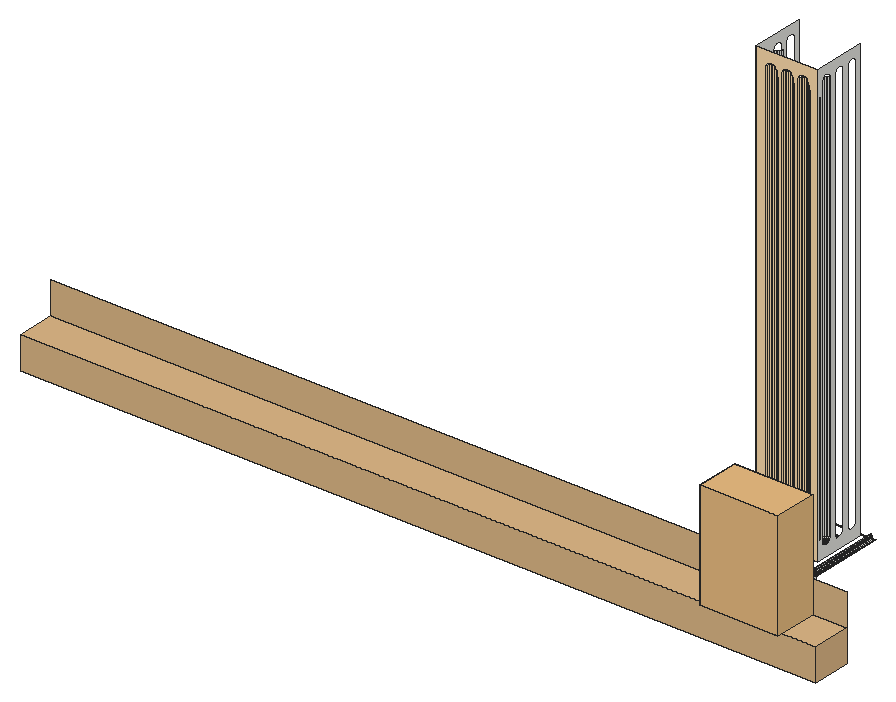
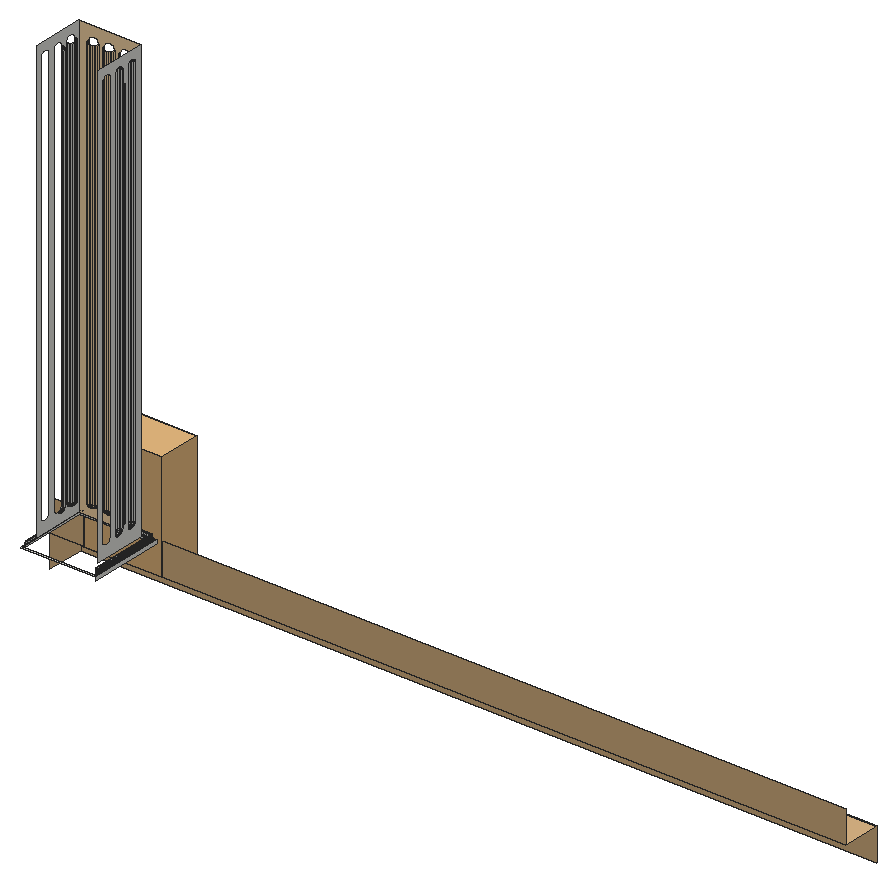
# SketchUp Ruby script. Lengths in inches.
U = 1.inch
M = Sketchup.active_model
def pt(a) = Geom::Point3d.new(a.map { |v| v * U })
def face(e, loops, mat)
  f = e.add_face(loops[0].map { |a| pt(a) })
  loops[1..].each { |l| e.add_face(l.map { |a| pt(a) }).erase! }
  f.material = f.back_material = mat if mat
  f
end
# faces: each face lists its corners as indices into pts; further lists are holes
def faces(e, pts, list, mat = nil) = list.each { |f| face(e, (f[0].is_a?(Array) ? f : [f]).map { |l| l.map { |i| pts[i] } }, mat) }
# xy, xz, yz: faces in a plane at the given z, y or x. An outline is a flat list of corners, or four numbers for a rectangle; further outlines are holes
def ring(l) = l.size == 4 ? [[l[0], l[1]], [l[2], l[1]], [l[2], l[3]], [l[0], l[3]]] : l.each_slice(2).to_a
def flat(e, list, mat, &to3) = list.each { |f| face(e, (f[0].is_a?(Array) ? f : [f]).map { |l| ring(l).map { |u, v| to3.(u, v) } }, mat) }
def xy(e, z, list, mat = nil) = flat(e, list, mat) { |x, y| [x, y, z] }
def xz(e, y, list, mat = nil) = flat(e, list, mat) { |x, z| [x, y, z] }
def yz(e, x, list, mat = nil) = flat(e, list, mat) { |y, z| [x, y, z] }
def lines(e, pts, list) = list.each { |a, b| e.add_line(pt(pts[a]), pt(pts[b])) }
# prism: a flat outline (further loops are holes) pulled along v
def prism(e, loops, v, mat = nil)
  f = face(e, loops, mat); d = Geom::Vector3d.new(v.map { |x| x * U })
  f.pushpull(f.normal.samedirection?(d) ? d.length : -d.length)
end
def box(e, o, s, mat = nil) = prism(e, [[o, [o[0] + s[0], o[1], o[2]], [o[0] + s[0], o[1] + s[1], o[2]], [o[0], o[1] + s[1], o[2]]]], [0, 0, s[2]], mat)
def at(x, y, z, deg = 0) = Geom::Transformation.translation(pt([x, y, z])) * Geom::Transformation.rotation(ORIGIN, Z_AXIS, deg.degrees)
def axes(o, x, y, z) = Geom::Transformation.new([*x, 0, *y, 0, *z, 0, *pt(o).to_a, 1])
def part(name) = M.definitions.add(name)
# library, detail: a bought-in or finely detailed component or shape, given as its bounding box
def library(name, o, s) = part(name).tap { |d| box(d.entities, o, s) }
def detail(e, o, s) = box(e.add_group.entities, o, s)
def put(e, d, t, mat = nil) = e.add_instance(d, t).tap { |i| i.material = mat if mat }
def group(e, t, mat = nil) = e.add_group.tap { |g| g.transformation = t; g.material = mat if mat }.entities
root = M.entities
M.materials.add("[0033_NavajoWhite]").color = [255, 222, 173]
M.materials.add("[0036_BurlyWood]").color = [222, 184, 135]
c1 = library("Flower+pot",[-3.29,-4.11,0],[8.25,8.08,16.09])
xy(root,6,[[103.43,0,251.04,7.125]],"[0036_BurlyWood]")
xy(root,12.13,[[[230.94,7.58,244.97,21.61],[231.11,7.74,244.81,21.44]]])
xz(root,0,[[103.43,0,251.04,6]],"[0036_BurlyWood]")
xz(root,7.125,[[103.43,6,251.04,12]],"[0036_BurlyWood]")
xz(root,7.58,[[230.94,11.46,244.97,12.13]])
xz(root,8.1,[[231.46,12.13,244.45,13.02],[231.46,13.02,244.45,13.17]])
xz(root,9.67,[[[232.25,13.17,243.67,94.95],[235.01,14.97,234.75,15,234.51,15.09,234.31,15.24,234.15,15.42,234.05,15.64,234.02,15.875,234.02,92.25,234.05,92.48,234.15,92.7,234.31,92.89,234.51,93.03,234.75,93.12,235.01,93.15,235.26,93.12,235.5,93.03,235.7,92.89,235.86,92.7,235.96,92.48,235.99,92.25,235.99,15.875,235.96,15.64,235.86,15.42,235.7,15.24,235.5,15.09,235.26,15],[240.91,14.97,240.66,15,240.42,15.09,240.22,15.24,240.06,15.42,239.96,15.64,239.93,15.875,239.93,92.25,239.96,92.48,240.06,92.7,240.22,92.89,240.42,93.03,240.66,93.12,240.91,93.15,241.17,93.12,241.4,93.03,241.61,92.89,241.76,92.7,241.86,92.48,241.9,92.25,241.9,15.875,241.86,15.64,241.76,15.42,241.61,15.24,241.4,15.09,241.17,15],[237.96,14.97,237.7,15,237.47,15.09,237.26,15.24,237.11,15.42,237.01,15.64,236.97,15.875,236.97,92.25,237.01,92.48,237.11,92.7,237.26,92.89,237.47,93.03,237.7,93.12,237.96,93.15,238.21,93.12,238.45,93.03,238.65,92.89,238.8125,92.7,238.91,92.48,238.94,92.25,238.94,15.875,238.91,15.64,238.8125,15.42,238.65,15.24,238.45,15.09,238.21,15]]],"[0033_NavajoWhite]")
yz(root,230.94,[[7.58,11.46,21.61,12.13]])
yz(root,231.46,[[8.1,12.13,21.09,13.02],[8.1,13.02,21.09,13.17]])
yz(root,232.25,[[[9.67,13.17,19.51,94.95],[17.55,15.23,17.8,15.27,18.04,15.36,18.24,15.5,18.4,15.69,18.5,15.9,18.53,16.14,18.53,92.51,18.5,92.74,18.4,92.96,18.24,93.15,18.04,93.29,17.8,93.38,17.55,93.41,17.29,93.38,17.05,93.29,16.85,93.15,16.69,92.96,16.59,92.74,16.5625,92.51,16.5625,16.14,16.59,15.9,16.69,15.69,16.85,15.5,17.05,15.36,17.29,15.27],[14.59,15.23,14.85,15.27,15.08,15.36,15.29,15.5,15.44,15.69,15.54,15.9,15.58,16.14,15.58,92.51,15.54,92.74,15.44,92.96,15.29,93.15,15.08,93.29,14.85,93.38,14.59,93.41,14.34,93.38,14.1,93.29,13.9,93.15,13.74,92.96,13.64,92.74,13.61,92.51,13.61,16.14,13.64,15.9,13.74,15.69,13.9,15.5,14.1,15.36,14.34,15.27],[11.64,15.23,11.89,15.27,12.13,15.36,12.34,15.5,12.49,15.69,12.59,15.9,12.625,16.14,12.625,92.51,12.59,92.74,12.49,92.96,12.34,93.15,12.13,93.29,11.89,93.38,11.64,93.41,11.39,93.38,11.15,93.29,10.94,93.15,10.79,92.96,10.6875,92.74,10.66,92.51,10.66,16.14,10.6875,15.9,10.79,15.69,10.94,15.5,11.15,15.36,11.39,15.27]]])
yz(root,243.67,[[[9.67,13.17,19.51,94.95],[17.55,15.23,17.29,15.27,17.05,15.36,16.85,15.5,16.69,15.69,16.59,15.9,16.5625,16.14,16.5625,92.51,16.59,92.74,16.69,92.96,16.85,93.15,17.05,93.29,17.29,93.38,17.55,93.41,17.8,93.38,18.04,93.29,18.24,93.15,18.4,92.96,18.5,92.74,18.53,92.51,18.53,16.14,18.5,15.9,18.4,15.69,18.24,15.5,18.04,15.36,17.8,15.27],[14.59,15.23,14.34,15.27,14.1,15.36,13.9,15.5,13.74,15.69,13.64,15.9,13.61,16.14,13.61,92.51,13.64,92.74,13.74,92.96,13.9,93.15,14.1,93.29,14.34,93.38,14.59,93.41,14.85,93.38,15.08,93.29,15.29,93.15,15.44,92.96,15.54,92.74,15.58,92.51,15.58,16.14,15.54,15.9,15.44,15.69,15.29,15.5,15.08,15.36,14.85,15.27],[11.64,15.23,11.39,15.27,11.15,15.36,10.94,15.5,10.79,15.69,10.6875,15.9,10.66,16.14,10.66,92.51,10.6875,92.74,10.79,92.96,10.94,93.15,11.15,93.29,11.39,93.38,11.64,93.41,11.89,93.38,12.13,93.29,12.34,93.15,12.49,92.96,12.59,92.74,12.625,92.51,12.625,16.14,12.59,15.9,12.49,15.69,12.34,15.5,12.13,15.36,11.89,15.27]]])
yz(root,244.45,[[8.1,12.13,21.09,13.02],[8.1,13.02,21.09,13.17]])
yz(root,251.04,[[0,0,7.125,6]],"[0036_BurlyWood]")
p = [[244.81,7.74,12.13],[244.78,7.78,12.15],[231.14,7.78,12.15],[231.11,7.74,12.13],[231.14,21.41,12.15],[231.11,21.44,12.13],
  [244.81,21.44,12.13],[244.78,21.41,12.15],[244.71,7.84,12.2],[231.2,7.84,12.2],[231.2,21.35,12.2],[244.71,21.35,12.2],
  [244.65,7.9,12.27],[231.26,7.9,12.27],[231.26,21.29,12.27],[244.65,21.29,12.27],[244.6,7.95,12.36],[231.32,7.95,12.36],
  [231.32,21.24,12.36],[244.6,21.24,12.36],[244.55,8,12.47],[231.36,8,12.47],[231.36,21.1875,12.47],[244.55,21.1875,12.47],
  [244.52,8.03,12.59],[231.4,8.03,12.59],[231.4,21.15,12.59],[244.52,21.15,12.59],[244.49,8.06,12.73],[231.43,8.06,12.73],
  [231.43,21.12,12.73],[244.49,21.12,12.73],[244.47,8.09,12.87],[231.45,8.09,12.87],[231.45,21.1,12.87],[244.47,21.1,12.87],
  [244.45,8.1,13.02],[231.46,8.1,13.02],[231.46,21.09,13.02],[244.45,21.09,13.02],[234.53,9.8,15.09],[234.51,9.67,15.09],
  [234.75,9.67,15],[234.76,9.74,15],[234.78,9.8,15],[234.58,9.92,15.09],[235.01,9.67,14.97],[234.83,9.85,15],
  [234.88,9.89,15],[234.94,9.92,15],[235.01,9.93,15],[235.25,9.74,15],[235.26,9.67,15],[235.23,9.8,15],
  [235.1875,9.85,15],[235.13,9.89,15],[235.07,9.92,15],[235.48,9.8,15.09],[235.43,9.92,15.09],[235.5,9.67,15.09],
  [237.48,9.8,15.09],[237.47,9.67,15.09],[237.7,9.67,15],[237.71,9.74,15],[237.74,9.8,15],[237.53,9.92,15.09],
  [237.96,9.67,14.97],[237.78,9.85,15],[237.83,9.89,15],[237.89,9.92,15],[237.96,9.93,15],[238.2,9.74,15],
  [238.21,9.67,15],[238.18,9.8,15],[238.14,9.85,15],[238.09,9.89,15],[238.02,9.92,15],[238.45,9.67,15.09],
  [238.43,9.8,15.09],[238.38,9.92,15.09],[240.4375,9.8,15.09],[240.42,9.67,15.09],[240.66,9.67,15],[240.67,9.74,15],
  [240.69,9.8,15],[240.48,9.92,15.09],[240.91,9.67,14.97],[240.73,9.85,15],[240.78,9.89,15],[240.85,9.92,15],
  [240.91,9.93,15],[241.16,9.74,15],[241.17,9.67,15],[241.13,9.8,15],[241.09,9.85,15],[241.04,9.89,15],
  [240.98,9.92,15],[241.39,9.8,15.09],[241.34,9.92,15.09],[241.4,9.67,15.09],[234.66,10.02,15.09],[235.35,10.02,15.09],
  [237.61,10.02,15.09],[238.31,10.02,15.09],[240.5625,10.02,15.09],[241.26,10.02,15.09],[234.76,10.1,15.09],[234.88,10.15,15.09],
  [235.01,10.16,15.09],[235.13,10.15,15.09],[235.25,10.1,15.09],[237.71,10.1,15.09],[237.83,10.15,15.09],[237.96,10.16,15.09],
  [238.2,10.1,15.09],[238.09,10.15,15.09],[240.67,10.1,15.09],[240.78,10.15,15.09],[240.91,10.16,15.09],[241.04,10.15,15.09],
  [241.16,10.1,15.09],[234.33,9.85,15.24],[234.31,9.67,15.24],[235.7,9.67,15.24],[235.68,9.85,15.24],[237.29,9.85,15.24],
  [237.26,9.67,15.24],[238.65,9.67,15.24],[238.63,9.85,15.24],[240.24,9.85,15.24],[240.22,9.67,15.24],[241.61,9.67,15.24],
  [241.58,9.85,15.24],[234.4,10.02,15.24],[235.61,10.02,15.24],[237.36,10.02,15.24],[238.5625,10.02,15.24],[240.31,10.02,15.24],
  [241.51,10.02,15.24],[234.51,10.16,15.24],[235.5,10.16,15.24],[237.47,10.16,15.24],[238.45,10.16,15.24],[240.42,10.16,15.24],
  [241.4,10.16,15.24],[234.66,10.27,15.24],[235.35,10.27,15.24],[237.61,10.27,15.24],[238.31,10.27,15.24],[240.5625,10.27,15.24],
  [241.26,10.27,15.24],[234.83,10.34,15.24],[235.01,10.37,15.24],[235.1875,10.34,15.24],[237.78,10.34,15.24],[237.96,10.37,15.24],
  [238.14,10.34,15.24],[240.73,10.34,15.24],[240.91,10.37,15.24],[241.09,10.34,15.24],[234.18,9.89,15.42],[234.15,9.67,15.42],
  [235.86,9.67,15.42],[235.83,9.89,15.42],[237.14,9.89,15.42],[237.11,9.67,15.42],[238.8125,9.67,15.42],[238.78,9.89,15.42],
  [240.09,9.89,15.42],[240.06,9.67,15.42],[241.76,9.67,15.42],[241.73,9.89,15.42],[234.27,10.1,15.42],[235.74,10.1,15.42],
  [237.22,10.1,15.42],[238.7,10.1,15.42],[240.17,10.1,15.42],[241.65,10.1,15.42],[234.4,10.27,15.42],[235.61,10.27,15.42],
  [237.36,10.27,15.42],[238.5625,10.27,15.42],[240.31,10.27,15.42],[241.51,10.27,15.42],[234.58,10.41,15.42],[235.43,10.41,15.42],
  [237.53,10.41,15.42],[238.38,10.41,15.42],[240.48,10.41,15.42],[241.34,10.41,15.42],[234.78,10.49,15.42],[235.01,10.52,15.42],
  [235.23,10.49,15.42],[237.74,10.49,15.42],[237.96,10.52,15.42],[238.18,10.49,15.42],[240.69,10.49,15.42],[240.91,10.52,15.42],
  [241.13,10.49,15.42],[232.32,11.39,15.27],[232.25,11.64,15.23],[232.25,11.39,15.27],[232.38,11.42,15.27],[232.43,11.46,15.27],
  [243.6,11.39,15.27],[243.67,11.64,15.23],[243.54,11.42,15.27],[243.49,11.46,15.27],[243.67,11.39,15.27],[232.47,11.51,15.27],
  [232.5,11.57,15.27],[243.45,11.51,15.27],[243.42,11.57,15.27],[232.5,11.64,15.27],[232.5,11.71,15.27],[232.47,11.77,15.27],
  [232.43,11.82,15.27],[232.38,11.86,15.27],[232.32,11.89,15.27],[232.25,11.89,15.27],[243.41,11.64,15.27],[243.42,11.71,15.27],
  [243.45,11.77,15.27],[243.49,11.82,15.27],[243.54,11.86,15.27],[243.6,11.89,15.27],[243.67,11.89,15.27],[232.32,14.35,15.27],
  [232.25,14.59,15.23],[232.25,14.34,15.27],[232.38,14.37,15.27],[243.6,14.35,15.27],[243.67,14.59,15.23],[243.54,14.37,15.27],
  [243.67,14.34,15.27],[232.43,14.41,15.27],[232.47,14.47,15.27],[243.49,14.41,15.27],[243.45,14.47,15.27],[232.5,14.53,15.27],
  [232.5,14.59,15.27],[243.42,14.53,15.27],[243.41,14.59,15.27],[232.25,11.15,15.36],[232.38,11.16,15.36],[243.54,11.16,15.36],
  [243.67,11.15,15.36],[232.5,11.21,15.36],[232.6,11.29,15.36],[243.42,11.21,15.36],[243.32,11.29,15.36],[232.68,11.39,15.36],
  [243.24,11.39,15.36],[232.73,11.51,15.36],[243.19,11.51,15.36],[232.74,11.64,15.36],[243.17,11.64,15.36],[232.73,11.77,15.36],
  [243.19,11.77,15.36],[232.68,11.89,15.36],[243.24,11.89,15.36],[232.6,11.99,15.36],[232.5,12.07,15.36],[243.32,11.99,15.36],
  [243.42,12.07,15.36],[232.38,12.12,15.36],[232.25,12.13,15.36],[243.54,12.12,15.36],[243.67,12.13,15.36],[232.25,14.1,15.36],
  [232.38,14.12,15.36],[232.5,14.17,15.36],[243.54,14.12,15.36],[243.42,14.17,15.36],[243.67,14.1,15.36],[232.6,14.24,15.36],
  [232.68,14.35,15.36],[243.32,14.24,15.36],[243.24,14.35,15.36],[232.73,14.47,15.36],[243.19,14.47,15.36],[232.74,14.59,15.36],
  [243.17,14.59,15.36],[234.09,9.92,15.64],[234.05,9.67,15.64],[235.96,9.67,15.64],[235.92,9.92,15.64],[237.04,9.92,15.64],
  [237.01,9.67,15.64],[238.91,9.67,15.64],[238.875,9.92,15.64],[239.99,9.92,15.64],[239.96,9.67,15.64],[241.86,9.67,15.64],
  [241.83,9.92,15.64],[234.18,10.15,15.64],[235.83,10.15,15.64],[237.14,10.15,15.64],[238.78,10.15,15.64],[240.09,10.15,15.64],
  [241.73,10.15,15.64],[234.33,10.34,15.64],[235.68,10.34,15.64],[237.29,10.34,15.64],[238.63,10.34,15.64],[240.24,10.34,15.64],
  [241.58,10.34,15.64],[234.53,10.49,15.64],[235.48,10.49,15.64],[237.48,10.49,15.64],[238.43,10.49,15.64],[240.4375,10.49,15.64],
  [241.39,10.49,15.64],[234.76,10.59,15.64],[235.25,10.59,15.64],[237.71,10.59,15.64],[238.2,10.59,15.64],[240.67,10.59,15.64],
  [241.16,10.59,15.64],[235.01,10.62,15.64],[237.96,10.62,15.64],[240.91,10.62,15.64],[232.25,10.94,15.5],[232.43,10.97,15.5],
  [243.49,10.97,15.5],[243.67,10.94,15.5],[232.6,11.04,15.5],[232.74,11.15,15.5],[243.32,11.04,15.5],[243.17,11.15,15.5],
  [232.85,11.29,15.5],[243.0625,11.29,15.5],[232.92,11.46,15.5],[242.99,11.46,15.5],[232.95,11.64,15.5],[242.97,11.64,15.5],
  [232.92,11.82,15.5],[242.99,11.82,15.5],[232.85,11.99,15.5],[243.0625,11.99,15.5],[232.74,12.13,15.5],[243.17,12.13,15.5],
  [232.6,12.24,15.5],[243.32,12.24,15.5],[232.43,12.3125,15.5],[232.25,12.34,15.5],[243.49,12.3125,15.5],[243.67,12.34,15.5],
  [232.25,13.9,15.5],[232.43,13.92,15.5],[232.6,13.99,15.5],[243.49,13.92,15.5],[243.32,13.99,15.5],[243.67,13.9,15.5],
  [232.74,14.1,15.5],[243.17,14.1,15.5],[232.85,14.24,15.5],[243.0625,14.24,15.5],[232.92,14.41,15.5],[242.99,14.41,15.5],
  [232.95,14.59,15.5],[242.97,14.59,15.5],[232.25,10.79,15.69],[232.47,10.82,15.69],[232.68,10.9,15.69],[243.45,10.82,15.69],
  [243.24,10.9,15.69],[243.67,10.79,15.69],[232.85,11.04,15.69],[243.0625,11.04,15.69],[232.99,11.21,15.69],[242.93,11.21,15.69],
  [233.07,11.42,15.69],[242.84,11.42,15.69],[233.1,11.64,15.69],[242.81,11.64,15.69],[233.07,11.86,15.69],[242.84,11.86,15.69],
  [232.99,12.07,15.69],[242.93,12.07,15.69],[232.85,12.24,15.69],[243.0625,12.24,15.69],[232.68,12.38,15.69],[243.24,12.38,15.69],
  [232.47,12.46,15.69],[243.45,12.46,15.69],[232.25,12.49,15.69],[243.67,12.49,15.69],[232.25,13.74,15.69],[232.47,13.77,15.69],
  [243.45,13.77,15.69],[243.67,13.74,15.69],[232.68,13.85,15.69],[243.24,13.85,15.69],[232.85,13.99,15.69],[243.0625,13.99,15.69],
  [232.99,14.17,15.69],[242.93,14.17,15.69],[233.07,14.37,15.69],[242.84,14.37,15.69],[233.1,14.59,15.69],[242.81,14.59,15.69],
  [234.05,9.93,15.875],[234.02,9.67,15.875],[235.99,9.67,15.875],[235.96,9.93,15.875],[237.01,9.93,15.875],[236.97,9.67,15.875],
  [238.94,9.67,15.875],[238.91,9.93,15.875],[239.96,9.93,15.875],[239.93,9.67,15.875],[241.9,9.67,15.875],[241.86,9.93,15.875],
  [234.15,10.16,15.875],[235.86,10.16,15.875],[237.11,10.16,15.875],[238.8125,10.16,15.875],[240.06,10.16,15.875],[241.76,10.16,15.875],
  [234.31,10.37,15.875],[235.7,10.37,15.875],[237.26,10.37,15.875],[238.65,10.37,15.875],[240.22,10.37,15.875],[241.61,10.37,15.875],
  [234.51,10.52,15.875],[235.5,10.52,15.875],[237.47,10.52,15.875],[238.45,10.52,15.875],[240.42,10.52,15.875],[241.4,10.52,15.875],
  [234.75,10.62,15.875],[235.26,10.62,15.875],[237.7,10.62,15.875],[238.21,10.62,15.875],[240.66,10.62,15.875],[241.17,10.62,15.875],
  [235.01,10.66,15.875],[237.96,10.66,15.875],[240.91,10.66,15.875],[232.25,10.6875,15.9],[232.5,10.72,15.9],[232.73,10.82,15.9],
  [243.42,10.72,15.9],[243.19,10.82,15.9],[243.67,10.6875,15.9],[232.92,10.97,15.9],[242.99,10.97,15.9],[233.07,11.16,15.9],
  [242.84,11.16,15.9],[233.17,11.39,15.9],[242.75,11.39,15.9],[233.2,11.64,15.9],[242.72,11.64,15.9],[233.17,11.89,15.9],
  [242.75,11.89,15.9],[233.07,12.12,15.9],[242.84,12.12,15.9],[232.92,12.3125,15.9],[242.99,12.3125,15.9],[232.73,12.46,15.9],
  [243.19,12.46,15.9],[232.5,12.56,15.9],[243.42,12.56,15.9],[232.25,12.59,15.9],[243.67,12.59,15.9],[232.25,13.64,15.9],
  [232.5,13.67,15.9],[243.42,13.67,15.9],[243.67,13.64,15.9],[232.73,13.77,15.9],[243.19,13.77,15.9],[232.92,13.92,15.9],
  [242.99,13.92,15.9],[233.07,14.12,15.9],[242.84,14.12,15.9],[233.17,14.35,15.9],[242.75,14.35,15.9],[233.2,14.59,15.9],
  [242.72,14.59,15.9],[234.05,9.93,92.25],[234.02,9.67,92.25],[235.99,9.67,92.25],[235.96,9.93,92.25],[237.01,9.93,92.25],
  [236.97,9.67,92.25],[238.94,9.67,92.25],[238.91,9.93,92.25],[239.96,9.93,92.25],[239.93,9.67,92.25],[241.9,9.67,92.25],
  [241.86,9.93,92.25],[234.15,10.16,92.25],[235.86,10.16,92.25],[237.11,10.16,92.25],[238.8125,10.16,92.25],[240.06,10.16,92.25],
  [241.76,10.16,92.25],[234.31,10.37,92.25],[235.7,10.37,92.25],[237.26,10.37,92.25],[238.65,10.37,92.25],[240.22,10.37,92.25],
  [241.61,10.37,92.25],[234.51,10.52,92.25],[235.5,10.52,92.25],[237.47,10.52,92.25],[238.45,10.52,92.25],[240.42,10.52,92.25],
  [241.4,10.52,92.25],[234.75,10.62,92.25],[235.26,10.62,92.25],[237.7,10.62,92.25],[238.21,10.62,92.25],[240.66,10.62,92.25],
  [241.17,10.62,92.25],[235.01,10.66,92.25],[237.96,10.66,92.25],[240.91,10.66,92.25],[232.25,10.66,16.14],[232.5,10.6875,16.14],
  [232.74,10.79,16.14],[243.41,10.6875,16.14],[243.17,10.79,16.14],[243.67,10.66,16.14],[232.95,10.94,16.14],[242.97,10.94,16.14],
  [233.1,11.15,16.14],[242.81,11.15,16.14],[233.2,11.39,16.14],[242.72,11.39,16.14],[233.23,11.64,16.14],[242.68,11.64,16.14],
  [233.2,11.89,16.14],[242.72,11.89,16.14],[233.1,12.13,16.14],[242.81,12.13,16.14],[232.95,12.34,16.14],[242.97,12.34,16.14],
  [232.74,12.49,16.14],[243.17,12.49,16.14],[232.5,12.59,16.14],[243.41,12.59,16.14],[232.25,12.625,16.14],[243.67,12.625,16.14],
  [232.25,13.61,16.14],[232.5,13.64,16.14],[232.74,13.74,16.14],[243.41,13.64,16.14],[243.17,13.74,16.14],[243.67,13.61,16.14],
  [232.95,13.9,16.14],[242.97,13.9,16.14],[233.1,14.1,16.14],[242.81,14.1,16.14],[233.2,14.34,16.14],[242.72,14.34,16.14],
  [233.23,14.59,16.14],[242.68,14.59,16.14],[232.25,10.66,92.51],[232.5,10.6875,92.51],[232.74,10.79,92.51],[243.17,10.79,92.51],
  [243.41,10.6875,92.51],[243.67,10.66,92.51],[232.95,10.94,92.51],[242.97,10.94,92.51],[233.1,11.15,92.51],[242.81,11.15,92.51],
  [233.2,11.39,92.51],[242.72,11.39,92.51],[233.23,11.64,92.51],[242.68,11.64,92.51],[233.2,11.89,92.51],[242.72,11.89,92.51],
  [233.1,12.13,92.51],[242.81,12.13,92.51],[232.95,12.34,92.51],[242.97,12.34,92.51],[232.74,12.49,92.51],[243.17,12.49,92.51],
  [232.5,12.59,92.51],[243.41,12.59,92.51],[232.25,12.625,92.51],[243.67,12.625,92.51],[232.25,13.61,92.51],[232.5,13.64,92.51],
  [232.74,13.74,92.51],[243.17,13.74,92.51],[243.41,13.64,92.51],[243.67,13.61,92.51],[232.95,13.9,92.51],[242.97,13.9,92.51],
  [233.1,14.1,92.51],[242.81,14.1,92.51],[233.2,14.34,92.51],[242.72,14.34,92.51],[233.23,14.59,92.51],[242.68,14.59,92.51],
  [245.1,7.45,11.45],[245.14,7.41,11.4],[245.18,7.37,11.33]]
faces(root,p,[[0,1,2,3],[2,4,5,3],[0,6,7,1],[1,8,9,2],[9,10,4,2],[1,7,11,8],[8,12,13,9],[13,14,10,9],
  [8,11,15,12],[12,16,17,13],[17,18,14,13],[12,15,19,16],[16,20,21,17],[21,22,18,17],[16,19,23,20],[20,24,25,21],
  [25,26,22,21],[20,23,27,24],[24,28,29,25],[29,30,26,25],[24,27,31,28],[28,32,33,29],[33,34,30,29],[28,31,35,32],
  [32,36,37,33],[37,38,34,33],[32,35,39,36],[199,200,201],[200,199,202],[200,202,203],[204,205,206],[206,205,207],
  [205,204,208],[200,203,209],[200,209,210],[207,205,211],[211,205,212],[200,210,213],[200,213,214],[200,214,215],
  [200,215,216],[200,216,217],[200,217,218],[218,219,200],[212,205,220],[220,205,221],[221,205,222],[222,205,223],
  [223,205,224],[224,205,225],[226,225,205],[227,228,229],[228,227,230],[231,232,233],[232,231,234],[228,230,235],
  [228,235,236],[237,232,238],[233,232,237],[228,236,239],[228,239,240],[238,232,241],[241,232,242],[199,201,243,244],
  [208,204,245,246],[199,244,247,202],[202,247,248,203],[249,206,207,250],[245,204,206,249],[203,248,251,209],[250,207,211,252],[209,251,253,210],
  [252,211,212,254],[210,253,255,213],[254,212,220,256],[213,255,257,214],[256,220,221,258],[214,257,259,215],[258,221,222,260],[215,259,261,216],
  [216,261,262,217],[260,222,223,263],[263,223,224,264],[265,266,219,218],[217,262,265,218],[264,224,225,267],[268,267,225,226],[227,229,269,270],
  [227,270,271,230],[272,231,233,273],[234,231,272,274],[230,271,275,235],[235,275,276,236],[277,237,238,278],[273,233,237,277],[236,276,279,239],
  [278,238,241,280],[239,279,281,240],[280,241,242,282],[244,243,322,323],[246,245,324,325],[244,323,326,247],[247,326,327,248],[328,249,250,329],
  [324,245,249,328],[248,327,330,251],[329,250,252,331],[251,330,332,253],[331,252,254,333],[253,332,334,255],[333,254,256,335],[255,334,336,257],
  [335,256,258,337],[257,336,338,259],[337,258,260,339],[259,338,340,261],[339,260,263,341],[261,340,342,262],[341,263,264,343],[344,345,266,265],
  [262,342,344,265],[343,264,267,346],[347,346,267,268],[270,269,348,349],[270,349,350,271],[351,272,273,352],[274,272,351,353],[271,350,354,275],
  [352,273,277,355],[275,354,356,276],[355,277,278,357],[276,356,358,279],[357,278,280,359],[279,358,360,281],[359,280,282,361],[323,322,362,363],
  [323,363,364,326],[365,324,328,366],[325,324,365,367],[326,364,368,327],[366,328,329,369],[327,368,370,330],[369,329,331,371],[330,370,372,332],
  [371,331,333,373],[332,372,374,334],[373,333,335,375],[334,374,376,336],[375,335,337,377],[336,376,378,338],[377,337,339,379],[338,378,380,340],
  [379,339,341,381],[340,380,382,342],[381,341,343,383],[342,382,384,344],[383,343,346,385],[384,386,345,344],[387,385,346,347],[349,348,388,389],
  [353,351,390,391],[349,389,392,350],[390,351,352,393],[350,392,394,354],[393,352,355,395],[354,394,396,356],[395,355,357,397],[356,396,398,358],
  [397,357,359,399],[358,398,400,360],[399,359,361,401],[363,362,441,442],[363,442,443,364],[444,365,366,445],[367,365,444,446],[364,443,447,368],
  [445,366,369,448],[368,447,449,370],[448,369,371,450],[370,449,451,372],[450,371,373,452],[372,451,453,374],[452,373,375,454],[374,453,455,376],
  [454,375,377,456],[376,455,457,378],[456,377,379,458],[378,457,459,380],[458,379,381,460],[380,459,461,382],[460,381,383,462],[382,461,463,384],
  [462,383,385,464],[463,465,386,384],[466,464,385,387],[389,388,467,468],[391,390,469,470],[389,468,471,392],[469,390,393,472],[392,471,473,394],
  [472,393,395,474],[394,473,475,396],[474,395,397,476],[396,475,477,398],[476,397,399,478],[398,477,479,400],[478,399,401,480],[442,441,520,521],
  [442,521,522,443],[523,444,445,524],[446,444,523,525],[443,522,526,447],[524,445,448,527],[447,526,528,449],[527,448,450,529],[449,528,530,451],
  [529,450,452,531],[451,530,532,453],[531,452,454,533],[453,532,534,455],[533,454,456,535],[455,534,536,457],[535,456,458,537],[457,536,538,459],
  [537,458,460,539],[459,538,540,461],[539,460,462,541],[461,540,542,463],[541,462,464,543],[542,544,465,463],[545,543,464,466],[468,467,546,547],
  [468,547,548,471],[549,469,472,550],[470,469,549,551],[471,548,552,473],[550,472,474,553],[473,552,554,475],[553,474,476,555],[475,554,556,477],
  [555,476,478,557],[477,556,558,479],[557,478,480,559],[521,520,560,561],[522,521,561,562],[523,524,563,564],[525,523,564,565],[526,522,562,566],
  [524,527,567,563],[528,526,566,568],[527,529,569,567],[530,528,568,570],[529,531,571,569],[532,530,570,572],[531,533,573,571],[534,532,572,574],
  [533,535,575,573],[536,534,574,576],[535,537,577,575],[538,536,576,578],[537,539,579,577],[540,538,578,580],[539,541,581,579],[542,540,580,582],
  [541,543,583,581],[544,542,582,584],[543,545,585,583],[547,546,586,587],[548,547,587,588],[549,550,589,590],[551,549,590,591],[552,548,588,592],
  [550,553,593,589],[554,552,592,594],[553,555,595,593],[556,554,594,596],[555,557,597,595],[558,556,596,598],[557,559,599,597]])
faces(root,p,[[40,41,42,43],[44,45,40,43],[43,42,46],[46,44,43],[46,47,44],[46,48,47],[46,49,48],[46,50,49],
  [51,46,52],[46,51,53],[46,53,54],[46,54,55],[46,55,56],[46,56,50],[51,57,58,53],[51,52,59,57],
  [60,61,62,63],[64,65,60,63],[63,62,66],[66,64,63],[66,67,64],[66,68,67],[66,69,68],[66,70,69],
  [71,66,72],[66,71,73],[66,73,74],[66,74,75],[66,75,76],[66,76,70],[71,72,77,78],[71,78,79,73],
  [80,81,82,83],[84,85,80,83],[83,82,86],[86,84,83],[86,87,84],[86,88,87],[86,89,88],[86,90,89],
  [91,86,92],[86,91,93],[86,93,94],[86,94,95],[86,95,96],[86,96,90],[91,97,98,93],[91,92,99,97],
  [47,100,45,44],[53,58,101,54],[67,102,65,64],[73,79,103,74],[87,104,85,84],[93,98,105,94],[48,106,100,47],[49,107,106,48],
  [50,108,107,49],[56,109,108,50],[54,101,110,55],[55,110,109,56],[68,111,102,67],[69,112,111,68],[70,113,112,69],[75,114,115,76],
  [76,115,113,70],[74,103,114,75],[88,116,104,87],[89,117,116,88],[90,118,117,89],[96,119,118,90],[94,105,120,95],[95,120,119,96],
  [121,122,41,40],[57,59,123,124],[125,126,61,60],[78,77,127,128],[129,130,81,80],[97,99,131,132],[45,133,121,40],[57,124,134,58],
  [65,135,125,60],[78,128,136,79],[85,137,129,80],[97,132,138,98],[100,139,133,45],[58,134,140,101],[102,141,135,65],[79,136,142,103],
  [104,143,137,85],[98,138,144,105],[106,145,139,100],[101,140,146,110],[111,147,141,102],[103,142,148,114],[116,149,143,104],[105,144,150,120],
  [107,151,145,106],[108,152,151,107],[109,153,152,108],[110,146,153,109],[112,154,147,111],[113,155,154,112],[115,156,155,113],[114,148,156,115],
  [117,157,149,116],[118,158,157,117],[119,159,158,118],[120,150,159,119],[160,161,122,121],[124,123,162,163],[164,165,126,125],[128,127,166,167],
  [168,169,130,129],[132,131,170,171],[133,172,160,121],[124,163,173,134],[135,174,164,125],[128,167,175,136],[137,176,168,129],[132,171,177,138],
  [139,178,172,133],[134,173,179,140],[141,180,174,135],[136,175,181,142],[143,182,176,137],[138,177,183,144],[145,184,178,139],[140,179,185,146],
  [147,186,180,141],[142,181,187,148],[149,188,182,143],[144,183,189,150],[151,190,184,145],[152,191,190,151],[153,192,191,152],[146,185,192,153],
  [154,193,186,147],[155,194,193,154],[156,195,194,155],[148,187,195,156],[157,196,188,149],[158,197,196,157],[159,198,197,158],[150,189,198,159],
  [283,284,161,160],[163,162,285,286],[287,288,165,164],[167,166,289,290],[291,292,169,168],[171,170,293,294],[172,295,283,160],[163,286,296,173],
  [174,297,287,164],[167,290,298,175],[176,299,291,168],[171,294,300,177],[178,301,295,172],[173,296,302,179],[180,303,297,174],[175,298,304,181],
  [182,305,299,176],[177,300,306,183],[184,307,301,178],[179,302,308,185],[186,309,303,180],[181,304,310,187],[188,311,305,182],[183,306,312,189],
  [190,313,307,184],[185,308,314,192],[193,315,309,186],[187,310,316,195],[196,317,311,188],[189,312,318,198],[191,319,313,190],[192,314,319,191],
  [194,320,315,193],[195,316,320,194],[197,321,317,196],[198,318,321,197],[402,403,284,283],[286,285,404,405],[406,407,288,287],[290,289,408,409],
  [410,411,292,291],[294,293,412,413],[295,414,402,283],[286,405,415,296],[297,416,406,287],[290,409,417,298],[299,418,410,291],[294,413,419,300],
  [301,420,414,295],[296,415,421,302],[303,422,416,297],[298,417,423,304],[305,424,418,299],[300,419,425,306],[307,426,420,301],[302,421,427,308],
  [309,428,422,303],[304,423,429,310],[311,430,424,305],[306,425,431,312],[313,432,426,307],[308,427,433,314],[315,434,428,309],[310,429,435,316],
  [317,436,430,311],[312,431,437,318],[319,438,432,313],[314,433,438,319],[320,439,434,315],[316,435,439,320],[321,440,436,317],[318,437,440,321],
  [403,402,481,482],[405,404,483,484],[407,406,485,486],[409,408,487,488],[411,410,489,490],[413,412,491,492],[402,414,493,481],[415,405,484,494],
  [406,416,495,485],[417,409,488,496],[410,418,497,489],[419,413,492,498],[414,420,499,493],[421,415,494,500],[416,422,501,495],[423,417,496,502],
  [418,424,503,497],[425,419,498,504],[420,426,505,499],[427,421,500,506],[422,428,507,501],[429,423,502,508],[424,430,509,503],[431,425,504,510],
  [426,432,511,505],[433,427,506,512],[428,434,513,507],[435,429,508,514],[430,436,515,509],[437,431,510,516],[432,438,517,511],[438,433,512,517],
  [434,439,518,513],[439,435,514,518],[436,440,519,515],[440,437,516,519]],"[0033_NavajoWhite]")
lines(root,p,[[600,601],[601,602]])
put(root,c1,axes([236.02,3.16,6],[1.76453,0,0],[0,1,0],[0,0,1.24]))
